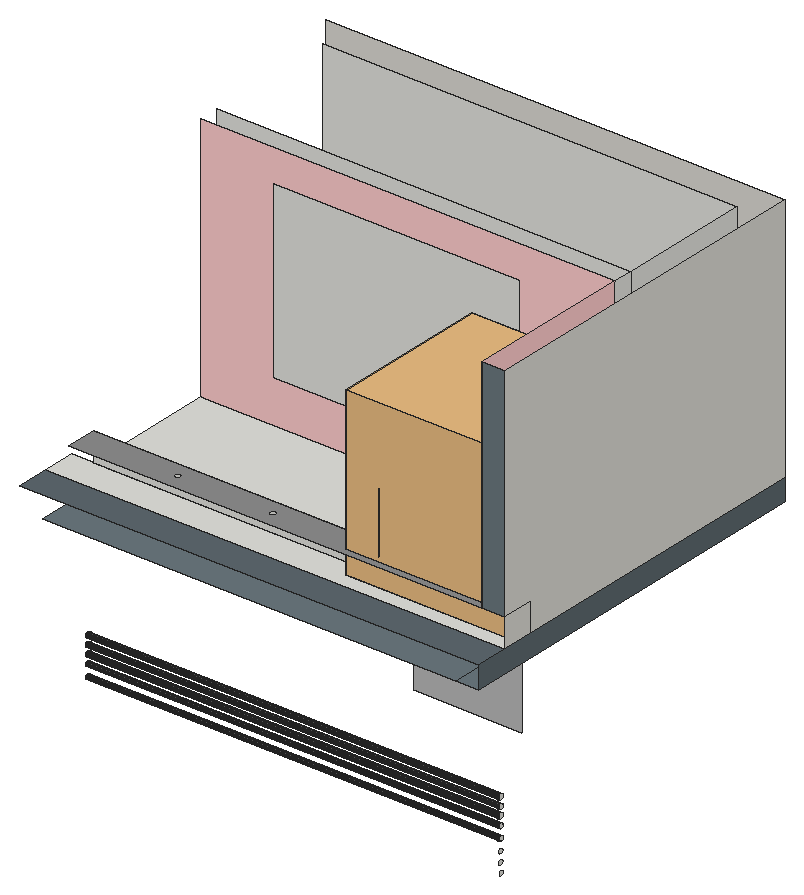
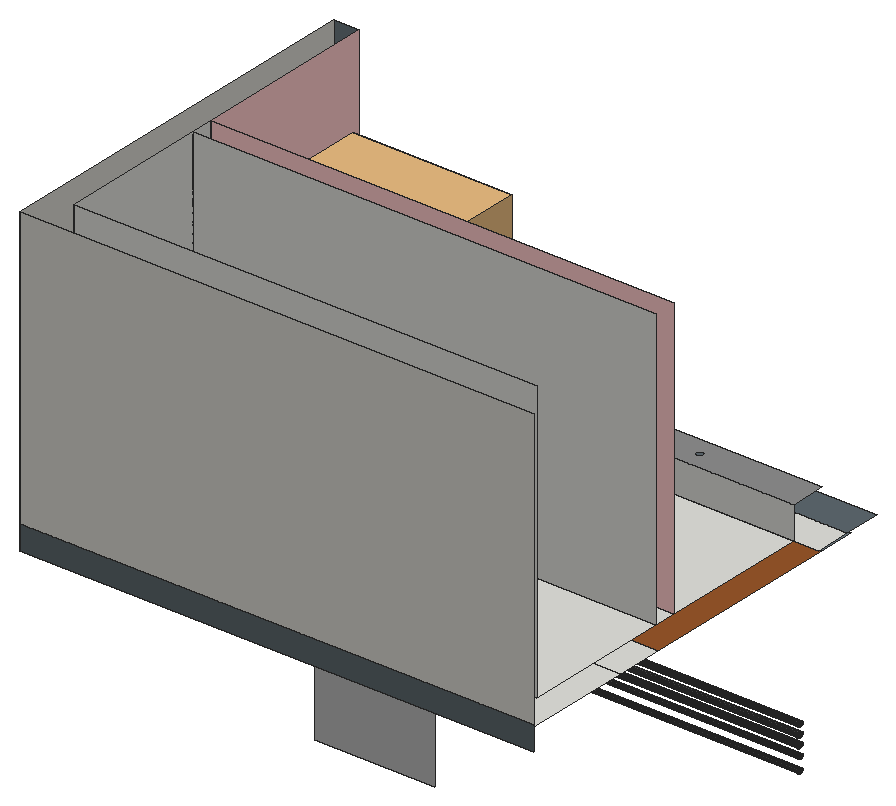
# SketchUp Ruby script. Lengths in inches.
U = 1.inch
M = Sketchup.active_model
def pt(a) = Geom::Point3d.new(a.map { |v| v * U })
def face(e, loops, mat)
  f = e.add_face(loops[0].map { |a| pt(a) })
  loops[1..].each { |l| e.add_face(l.map { |a| pt(a) }).erase! }
  f.material = f.back_material = mat if mat
  f
end
# faces: each face lists its corners as indices into pts; further lists are holes
def faces(e, pts, list, mat = nil) = list.each { |f| face(e, (f[0].is_a?(Array) ? f : [f]).map { |l| l.map { |i| pts[i] } }, mat) }
# xy, xz, yz: faces in a plane at the given z, y or x. An outline is a flat list of corners, or four numbers for a rectangle; further outlines are holes
def ring(l) = l.size == 4 ? [[l[0], l[1]], [l[2], l[1]], [l[2], l[3]], [l[0], l[3]]] : l.each_slice(2).to_a
def flat(e, list, mat, &to3) = list.each { |f| face(e, (f[0].is_a?(Array) ? f : [f]).map { |l| ring(l).map { |u, v| to3.(u, v) } }, mat) }
def xy(e, z, list, mat = nil) = flat(e, list, mat) { |x, y| [x, y, z] }
def xz(e, y, list, mat = nil) = flat(e, list, mat) { |x, z| [x, y, z] }
def yz(e, x, list, mat = nil) = flat(e, list, mat) { |y, z| [x, y, z] }
def lines(e, pts, list) = list.each { |a, b| e.add_line(pt(pts[a]), pt(pts[b])) }
# prism: a flat outline (further loops are holes) pulled along v
def prism(e, loops, v, mat = nil)
  f = face(e, loops, mat); d = Geom::Vector3d.new(v.map { |x| x * U })
  f.pushpull(f.normal.samedirection?(d) ? d.length : -d.length)
end
def box(e, o, s, mat = nil) = prism(e, [[o, [o[0] + s[0], o[1], o[2]], [o[0] + s[0], o[1] + s[1], o[2]], [o[0], o[1] + s[1], o[2]]]], [0, 0, s[2]], mat)
def at(x, y, z, deg = 0) = Geom::Transformation.translation(pt([x, y, z])) * Geom::Transformation.rotation(ORIGIN, Z_AXIS, deg.degrees)
def axes(o, x, y, z) = Geom::Transformation.new([*x, 0, *y, 0, *z, 0, *pt(o).to_a, 1])
def part(name) = M.definitions.add(name)
# library, detail: a bought-in or finely detailed component or shape, given as its bounding box
def library(name, o, s) = part(name).tap { |d| box(d.entities, o, s) }
def detail(e, o, s) = box(e.add_group.entities, o, s)
def put(e, d, t, mat = nil) = e.add_instance(d, t).tap { |i| i.material = mat if mat }
def group(e, t, mat = nil) = e.add_group.tap { |g| g.transformation = t; g.material = mat if mat }.entities
root = M.entities
M.materials.add("[Color A01]").color = [255, 204, 204]
M.materials.add("[Color M04]").color = [142, 142, 142]
M.materials.add("[Color M06]").color = [86, 86, 86]
M.materials.add("[Formica Speckled Grey]").color = [107, 120, 127]
M.materials.add("[Formica Speckled Grey]1").color = [94, 105, 111]
M.materials.add("[Mirror 01]").color = [185, 185, 185]
M.materials.add("[Terrazzo Tile Light]").color = [219, 217, 210]
M.materials.add("[Wood Cherry Original]").color = [152, 86, 42]
c1 = library("chau cay",[-24.34,-109.24,0],[56.46,62.58,79.69])
xy(root,157.1875,[[166.51,84,166.7,84.02,166.88,84.1,167.04,84.22,167.16,84.375,167.23,84.55,167.26,84.75,167.23,84.94,167.16,85.125,167.04,85.28,166.88,85.4,166.7,85.47,166.51,85.5,166.32,85.47,166.13,85.4,165.98,85.28,165.86,85.125,165.79,84.94,165.76,84.75,165.79,84.55,165.86,84.375,165.98,84.22,166.13,84.1,166.32,84.02]])
xy(root,195.875,[[202.95,77.29,209.59,113.38],[178.6,91.72,177.43,92.01,176.375,92.59,175.51,93.43,174.88,94.46,174.55,95.62,174.52,96.83,174.81,98,175.4,99.06,176.24,99.93,177.27,100.55,178.43,100.89,179.64,100.91,180.81,100.62,181.87,100.04,182.74,99.2,183.36,98.16,183.69,97,183.72,95.8,183.43,94.625,182.84,93.57,182.01,92.7,180.97,92.07,179.8125,91.74],[202.95,113.38,209.59,131.65],[80.125,131.65,202.95,143.96],[202.95,131.65,209.59,143.96],
  [80.125,143.96,202.95,174.55],[202.95,143.96,209.59,181.19]])
xy(root,195.875,[[80.125,67.6,202.95,77.29],[202.95,67.6,209.59,77.29]],"[Formica Speckled Grey]")
xy(root,195.875,[[[80.125,77.29,202.95,131.65],[178.6,91.72,179.8125,91.74,180.97,92.07,182.01,92.7,182.84,93.57,183.43,94.625,183.72,95.8,183.69,97,183.36,98.16,182.74,99.2,181.87,100.04,180.81,100.62,179.64,100.91,178.43,100.89,177.27,100.55,176.24,99.93,175.4,99.06,174.81,98,174.52,96.83,174.55,95.62,174.88,94.46,175.51,93.43,176.375,92.59,177.43,92.01],[137.04,91.72,138.25,91.74,139.41,92.07,140.44,92.7,141.28,93.57,141.86,94.625,142.15,95.8,142.13,97,141.8,98.16,141.17,99.2,140.3,100.04,139.25,100.62,138.07,100.91,136.87,100.89,135.71,100.55,134.67,99.93,133.84,99.06,133.25,98,132.96,96.83,132.98,95.62,133.32,94.46,133.94,93.43,134.8125,92.59,135.87,92.01],[102.79,91.72,104,91.74,105.16,92.07,106.19,92.7,107.03,93.57,107.61,94.625,107.9,95.8,107.88,97,107.55,98.16,106.92,99.2,106.05,100.04,105,100.62,103.82,100.91,102.62,100.89,101.46,100.55,100.42,99.93,99.59,99.06,99,98,98.71,96.83,98.73,95.62,99.07,94.46,99.69,93.43,100.5625,92.59,101.62,92.01]]],"[Wood Cherry Original]")
xy(root,202.375,[[73.48,77.29,209.59,86.77],[80.125,86.77,202.95,126.48],[80.125,126.48,202.95,132.38],[80.125,132.38,202.95,171.71]])
xy(root,202.375,[[73.48,67.6,209.59,77.29]],"[Formica Speckled Grey]1")
xy(root,210.9375,[[202.95,77.29,209.59,86.77],[169.66,81.17,169.4,81.21,169.16,81.31,168.95,81.46,168.8,81.67,168.7,81.91,168.66,82.17,168.7,82.43,168.8,82.67,168.95,82.88,169.16,83.04,169.4,83.14,169.66,83.17,169.92,83.14,170.16,83.04,170.37,82.88,170.53,82.67,170.625,82.43,170.66,82.17,170.625,81.91,170.53,81.67,170.37,81.46,170.16,81.31,169.92,81.21]])
xy(root,210.9375,[[[80.125,77.29,202.95,86.77],[108.66,81.17,108.4,81.21,108.16,81.31,107.95,81.46,107.8,81.67,107.7,81.91,107.66,82.17,107.7,82.43,107.8,82.67,107.95,82.88,108.16,83.04,108.4,83.14,108.66,83.17,108.92,83.14,109.16,83.04,109.37,82.88,109.53,82.67,109.625,82.43,109.66,82.17,109.625,81.91,109.53,81.67,109.37,81.46,109.16,81.31,108.92,81.21],[169.66,81.17,169.4,81.21,169.16,81.31,168.95,81.46,168.8,81.67,168.7,81.91,168.66,82.17,168.7,82.43,168.8,82.67,168.95,82.88,169.16,83.04,169.4,83.14,169.66,83.17,169.92,83.14,170.16,83.04,170.37,82.88,170.53,82.67,170.625,82.43,170.66,82.17,170.625,81.91,170.53,81.67,170.37,81.46,170.16,81.31,169.92,81.21],[136.97,81.17,136.71,81.21,136.47,81.31,136.27,81.46,136.11,81.67,136.01,81.91,135.97,82.17,136.01,82.43,136.11,82.67,136.27,82.88,136.47,83.04,136.71,83.14,136.97,83.17,137.23,83.14,137.47,83.04,137.68,82.88,137.84,82.67,137.9375,82.43,137.97,82.17,137.9375,81.91,137.84,81.67,137.68,81.46,137.47,81.31,137.23,81.21]]],"[Color M04]")
xz(root,77.29,[[202.95,210.9375,209.59,276.375]],"[Formica Speckled Grey]")
xz(root,86.77,[[80.125,202.375,202.95,210.9375],[202.95,202.375,209.59,210.9375]])
xz(root,126.48,[[[80.125,202.375,202.95,276.375],[101.56,215.09,174.81,266.84]]],"[Color A01]")
xz(root,131.65,[[139.18,142.9,171.11,185.91]],"[Mirror 01]")
xz(root,132.38,[[80.125,202.375,202.95,276.375]])
xz(root,171.71,[[80.125,202.375,202.95,276.375]])
xz(root,181.19,[[73.48,195.875,209.59,202.375]],"[Formica Speckled Grey]1")
xz(root,181.19,[[73.48,202.375,209.59,276.375]],"[Terrazzo Tile Light]")
yz(root,202.95,[[84.31,136.76,84.47,136.78,84.62,136.84,84.75,136.94,84.85,137.07,84.91,137.22,84.93,137.39,84.91,137.55,84.85,137.7,84.75,137.83,84.62,137.93,84.47,137.99,84.31,138.01,84.15,137.99,84,137.93,83.87,137.83,83.77,137.7,83.7,137.55,83.68,137.39,83.7,137.22,83.77,137.07,83.87,136.94,84,136.84,84.15,136.78],[84.14,139.71,84.3,139.73,84.45,139.79,84.58,139.89,84.68,140.02,84.74,140.17,84.77,140.33,84.74,140.49,84.68,140.64,84.58,140.77,84.45,140.87,84.3,140.93,84.14,140.96,83.98,140.93,83.83,140.87,83.7,140.77,83.6,140.64,83.54,140.49,83.52,140.33,83.54,140.17,83.6,140.02,83.7,139.89,83.83,139.79,83.98,139.73],[84.14,142.77,84.3,142.79,84.45,142.85,84.58,142.95,84.68,143.08,84.74,143.23,84.77,143.39,84.74,143.56,84.68,143.71,84.58,143.84,84.45,143.93,84.3,144,84.14,144.02,83.98,144,83.83,143.93,83.7,143.84,83.6,143.71,83.54,143.56,83.52,143.39,83.54,143.23,83.6,143.08,83.7,142.95,83.83,142.85,83.98,142.79],[84.31,145.95,84.47,145.97,84.62,146.03,84.75,146.13,84.85,146.26,84.91,146.41,84.93,146.57,84.91,146.74,84.85,146.89,84.75,147.02,84.62,147.11,84.47,147.18,84.31,147.2,84.15,147.18,84,147.11,83.87,147.02,83.77,146.89,83.7,146.74,83.68,146.57,83.7,146.41,83.77,146.26,83.87,146.13,84,146.03,84.15,145.97],[84.31,149.39,84.47,149.41,84.62,149.47,84.75,149.57,84.85,149.7,84.91,149.85,84.93,150.01,84.91,150.17,84.85,150.32,84.75,150.45,84.62,150.55,84.47,150.61,84.31,150.64,84.15,150.61,84,150.55,83.87,150.45,83.77,150.32,83.7,150.17,83.68,150.01,83.7,149.85,83.77,149.7,83.87,149.57,84,149.47,84.15,149.41],
  [84.34,151.97,84.51,152,84.68,152.06,84.82,152.17,84.93,152.32,85,152.48,85.02,152.66,85,152.84,84.93,153,84.82,153.15,84.68,153.26,84.51,153.32,84.34,153.35,84.16,153.32,83.99,153.26,83.85,153.15,83.74,153,83.67,152.84,83.65,152.66,83.67,152.48,83.74,152.32,83.85,152.17,83.99,152.06,84.16,152],[84.34,154.47,84.51,154.5,84.68,154.56,84.82,154.67,84.93,154.82,85,154.98,85.02,155.16,85,155.34,84.93,155.5,84.82,155.65,84.68,155.76,84.51,155.82,84.34,155.85,84.16,155.82,83.99,155.76,83.85,155.65,83.74,155.5,83.67,155.34,83.65,155.16,83.67,154.98,83.74,154.82,83.85,154.67,83.99,154.56,84.16,154.5],[84.34,157.04,84.51,157.06,84.68,157.13,84.82,157.24,84.93,157.38,85,157.54,85.02,157.72,85,157.9,84.93,158.07,84.82,158.21,84.68,158.32,84.51,158.39,84.34,158.41,84.16,158.39,83.99,158.32,83.85,158.21,83.74,158.07,83.67,157.9,83.65,157.72,83.67,157.54,83.74,157.38,83.85,157.24,83.99,157.13,84.16,157.06],[126.48,202.375,132.38,276.375],[132.38,202.375,171.71,276.375]])
yz(root,202.95,[[[86.77,202.375,86.77,210.9375,77.29,210.9375,77.29,276.375,126.48,276.375,126.48,202.375],[82.17,234.08,82.42,234.11,82.67,234.21,82.875,234.37,83.03,234.58,83.13,234.82,83.17,235.08,83.13,235.34,83.03,235.58,82.875,235.79,82.67,235.94,82.42,236.04,82.17,236.08,81.91,236.04,81.67,235.94,81.46,235.79,81.3,235.58,81.2,235.34,81.17,235.08,81.2,234.82,81.3,234.58,81.46,234.37,81.67,234.21,81.91,234.11],[82.38,211.9,82.55,211.92,82.7,211.98,82.83,212.08,82.92,212.21,82.99,212.36,83.01,212.52,82.99,212.68,82.92,212.83,82.83,212.96,82.7,213.0625,82.55,213.125,82.38,213.15,82.22,213.125,82.07,213.0625,81.94,212.96,81.84,212.83,81.78,212.68,81.76,212.52,81.78,212.36,81.84,212.21,81.94,212.08,82.07,211.98,82.22,211.92],[82.38,228.4,82.55,228.42,82.7,228.48,82.83,228.58,82.92,228.71,82.99,228.86,83.01,229.02,82.99,229.18,82.92,229.33,82.83,229.46,82.7,229.5625,82.55,229.625,82.38,229.65,82.22,229.625,82.07,229.5625,81.94,229.46,81.84,229.33,81.78,229.18,81.76,229.02,81.78,228.86,81.84,228.71,81.94,228.58,82.07,228.48,82.22,228.42],[82.38,217.52,82.55,217.54,82.7,217.61,82.83,217.71,82.92,217.83,82.99,217.99,83.01,218.15,82.99,218.31,82.92,218.46,82.83,218.59,82.7,218.6875,82.55,218.75,82.38,218.77,82.22,218.75,82.07,218.6875,81.94,218.59,81.84,218.46,81.78,218.31,81.76,218.15,81.78,217.99,81.84,217.83,81.94,217.71,82.07,217.61,82.22,217.54],[82.38,225.9,82.55,225.92,82.7,225.98,82.83,226.08,82.92,226.21,82.99,226.36,83.01,226.52,82.99,226.68,82.92,226.83,82.83,226.96,82.7,227.0625,82.55,227.125,82.38,227.15,82.22,227.125,82.07,227.0625,81.94,226.96,81.84,226.83,81.78,226.68,81.76,226.52,81.78,226.36,81.84,226.21,81.94,226.08,82.07,225.98,82.22,225.92],[82.38,220.46,82.55,220.48,82.7,220.54,82.83,220.64,82.92,220.77,82.99,220.92,83.01,221.08,82.99,221.25,82.92,221.4,82.83,221.53,82.7,221.625,82.55,221.6875,82.38,221.71,82.22,221.6875,82.07,221.625,81.94,221.53,81.84,221.4,81.78,221.25,81.76,221.08,81.78,220.92,81.84,220.77,81.94,220.64,82.07,220.54,82.22,220.48],[82.38,223.27,82.55,223.29,82.7,223.36,82.83,223.46,82.92,223.58,82.99,223.74,83.01,223.9,82.99,224.06,82.92,224.21,82.83,224.34,82.7,224.4375,82.55,224.5,82.38,224.52,82.22,224.5,82.07,224.4375,81.94,224.34,81.84,224.21,81.78,224.06,81.76,223.9,81.78,223.74,81.84,223.58,81.94,223.46,82.07,223.36,82.22,223.29],[82.38,214.83,82.55,214.86,82.7,214.92,82.83,215.02,82.92,215.15,82.99,215.3,83.01,215.46,82.99,215.62,82.92,215.77,82.83,215.9,82.7,216,82.55,216.0625,82.38,216.08,82.22,216.0625,82.07,216,81.94,215.9,81.84,215.77,81.78,215.62,81.76,215.46,81.78,215.3,81.84,215.15,81.94,215.02,82.07,214.92,82.22,214.86],[82.38,230.9,82.55,230.92,82.7,230.98,82.83,231.08,82.92,231.21,82.99,231.36,83.01,231.52,82.99,231.68,82.92,231.83,82.83,231.96,82.7,232.0625,82.55,232.125,82.38,232.15,82.22,232.125,82.07,232.0625,81.94,231.96,81.84,231.83,81.78,231.68,81.76,231.52,81.78,231.36,81.84,231.21,81.94,231.08,82.07,230.98,82.22,230.92]]],"[Color A01]")
yz(root,209.59,[[67.6,195.875,181.19,202.375]],"[Formica Speckled Grey]1")
yz(root,209.59,[[77.29,202.375,86.77,210.9375],[86.77,202.375,181.19,202.375,181.19,276.375,77.29,276.375,77.29,210.9375,86.77,210.9375]],"[Terrazzo Tile Light]")
p = [[202.95,84,146.03],[202.95,83.87,146.13],[80.125,83.87,146.13],[80.125,84,146.03],[202.95,84.15,145.97],[80.125,84.15,145.97],
  [202.95,84.62,146.03],[202.95,84.47,145.97],[80.125,84.47,145.97],[80.125,84.62,146.03],[202.95,84.75,146.13],[80.125,84.75,146.13],
  [202.95,83.77,146.26],[80.125,83.77,146.26],[202.95,84.85,146.26],[80.125,84.85,146.26],[202.95,83.7,146.41],[80.125,83.7,146.41],
  [202.95,84.91,146.41],[80.125,84.91,146.41],[202.95,83.68,146.57],[80.125,83.68,146.57],[202.95,84.93,146.57],[80.125,84.93,146.57],
  [202.95,83.7,146.74],[80.125,83.7,146.74],[202.95,84.91,146.74],[80.125,84.91,146.74],[202.95,83.77,146.89],[80.125,83.77,146.89],
  [202.95,84.85,146.89],[80.125,84.85,146.89],[202.95,83.87,147.02],[80.125,83.87,147.02],[202.95,84.75,147.02],[80.125,84.75,147.02],
  [202.95,84,147.11],[80.125,84,147.11],[202.95,84.62,147.11],[80.125,84.62,147.11],[202.95,84.15,147.18],[80.125,84.15,147.18],
  [202.95,84.47,147.18],[80.125,84.47,147.18],[202.95,84.31,147.2],[80.125,84.31,147.2],[202.95,84.15,149.41],[202.95,84,149.47],
  [80.125,84,149.47],[80.125,84.15,149.41],[202.95,84.31,149.39],[80.125,84.31,149.39],[202.95,84.47,149.41],[80.125,84.47,149.41],
  [202.95,84.62,149.47],[80.125,84.62,149.47],[202.95,83.87,149.57],[80.125,83.87,149.57],[202.95,84.75,149.57],[80.125,84.75,149.57],
  [202.95,83.77,149.7],[80.125,83.77,149.7],[202.95,84.85,149.7],[80.125,84.85,149.7],[202.95,83.7,149.85],[80.125,83.7,149.85],
  [202.95,84.91,149.85],[80.125,84.91,149.85],[202.95,83.68,150.01],[80.125,83.68,150.01],[202.95,84.93,150.01],[80.125,84.93,150.01],
  [202.95,83.7,150.17],[80.125,83.7,150.17],[202.95,84.91,150.17],[80.125,84.91,150.17],[202.95,83.77,150.32],[80.125,83.77,150.32],
  [202.95,84.85,150.32],[80.125,84.85,150.32],[202.95,83.87,150.45],[80.125,83.87,150.45],[202.95,84.75,150.45],[80.125,84.75,150.45],
  [202.95,84,150.55],[80.125,84,150.55],[202.95,84.62,150.55],[80.125,84.62,150.55],[202.95,84.15,150.61],[80.125,84.15,150.61],
  [202.95,84.31,150.64],[80.125,84.31,150.64],[202.95,84.47,150.61],[80.125,84.47,150.61],[202.95,84.16,152],[202.95,83.99,152.06],
  [80.125,83.99,152.06],[80.125,84.16,152],[202.95,84.34,151.97],[80.125,84.34,151.97],[202.95,84.51,152],[80.125,84.51,152],
  [202.95,84.68,152.06],[80.125,84.68,152.06],[202.95,83.85,152.17],[80.125,83.85,152.17],[202.95,84.82,152.17],[80.125,84.82,152.17],
  [202.95,83.74,152.32],[80.125,83.74,152.32],[202.95,84.93,152.32],[80.125,84.93,152.32],[202.95,83.67,152.48],[80.125,83.67,152.48],
  [202.95,85,152.48],[80.125,85,152.48],[202.95,83.65,152.66],[80.125,83.65,152.66],[202.95,85.02,152.66],[80.125,85.02,152.66],
  [202.95,83.67,152.84],[80.125,83.67,152.84],[202.95,85,152.84],[80.125,85,152.84],[202.95,83.74,153],[80.125,83.74,153],
  [202.95,84.93,153],[80.125,84.93,153],[202.95,83.85,153.15],[80.125,83.85,153.15],[202.95,84.82,153.15],[80.125,84.82,153.15],
  [202.95,83.99,153.26],[80.125,83.99,153.26],[202.95,84.68,153.26],[80.125,84.68,153.26],[202.95,84.16,153.32],[80.125,84.16,153.32],
  [202.95,84.34,153.35],[80.125,84.34,153.35],[202.95,84.51,153.32],[80.125,84.51,153.32],[202.95,84.16,154.5],[202.95,83.99,154.56],
  [80.125,83.99,154.56],[80.125,84.16,154.5],[202.95,84.34,154.47],[80.125,84.34,154.47],[202.95,84.51,154.5],[80.125,84.51,154.5],
  [202.95,84.68,154.56],[80.125,84.68,154.56],[202.95,83.85,154.67],[80.125,83.85,154.67],[202.95,84.82,154.67],[80.125,84.82,154.67],
  [202.95,83.74,154.82],[80.125,83.74,154.82],[202.95,84.93,154.82],[80.125,84.93,154.82],[202.95,83.67,154.98],[80.125,83.67,154.98],
  [202.95,85,154.98],[80.125,85,154.98],[202.95,83.65,155.16],[80.125,83.65,155.16],[202.95,85.02,155.16],[80.125,85.02,155.16],
  [202.95,83.67,155.34],[80.125,83.67,155.34],[202.95,85,155.34],[80.125,85,155.34],[202.95,83.74,155.5],[80.125,83.74,155.5],
  [202.95,84.93,155.5],[80.125,84.93,155.5],[202.95,83.85,155.65],[80.125,83.85,155.65],[202.95,84.82,155.65],[80.125,84.82,155.65],
  [202.95,83.99,155.76],[80.125,83.99,155.76],[202.95,84.68,155.76],[80.125,84.68,155.76],[202.95,84.16,155.82],[80.125,84.16,155.82],
  [202.95,84.34,155.85],[80.125,84.34,155.85],[202.95,84.51,155.82],[80.125,84.51,155.82],[202.95,84.34,157.04],[202.95,84.16,157.06],
  [80.125,84.16,157.06],[80.125,84.34,157.04],[202.95,84.51,157.06],[80.125,84.51,157.06],[202.95,83.99,157.13],[202.95,83.85,157.24],
  [80.125,83.85,157.24],[80.125,83.99,157.13],[202.95,84.68,157.13],[80.125,84.68,157.13],[202.95,84.82,157.24],[80.125,84.82,157.24],
  [202.95,83.74,157.38],[80.125,83.74,157.38],[202.95,83.67,157.54],[80.125,83.67,157.54],[202.95,83.65,157.72],[80.125,83.65,157.72],
  [202.95,85.02,157.72],[202.95,85,157.54],[80.125,85,157.54],[80.125,85.02,157.72],[202.95,83.67,157.9],[80.125,83.67,157.9],
  [202.95,85,157.9],[80.125,85,157.9],[202.95,83.74,158.07],[80.125,83.74,158.07],[202.95,84.93,158.07],[80.125,84.93,158.07],
  [202.95,83.85,158.21],[80.125,83.85,158.21],[202.95,84.82,158.21],[80.125,84.82,158.21],[202.95,83.99,158.32],[80.125,83.99,158.32],
  [202.95,84.68,158.32],[80.125,84.68,158.32],[202.95,84.16,158.39],[80.125,84.16,158.39],[202.95,84.51,158.39],[80.125,84.51,158.39],
  [202.95,84.34,158.41],[80.125,84.34,158.41],[169.16,81.31,210.9375],[169.4,81.21,210.9375],[169.4,81.21,234.625],[169.16,81.31,234.625],
  [169.66,81.17,210.9375],[169.66,81.17,234.625],[169.92,81.21,210.9375],[169.92,81.21,234.625],[170.16,81.31,210.9375],[170.16,81.31,234.625],
  [168.95,81.46,210.9375],[168.95,81.46,234.625],[170.37,81.46,210.9375],[170.37,81.46,234.625],[168.8,81.67,210.9375],[168.8,81.67,234.625],
  [170.53,81.67,210.9375],[170.53,81.67,234.625],[168.7,81.91,210.9375],[168.7,81.91,234.625],[170.625,81.91,210.9375],[170.625,81.91,234.625],
  [168.66,82.17,210.9375],[168.66,82.17,234.625],[170.66,82.17,210.9375],[170.66,82.17,234.625],[168.7,82.43,210.9375],[168.7,82.43,234.625],
  [170.625,82.43,210.9375],[170.625,82.43,234.625],[168.8,82.67,210.9375],[168.8,82.67,234.625],[170.53,82.67,210.9375],[170.53,82.67,234.625],
  [168.95,82.88,210.9375],[168.95,82.88,234.625],[170.37,82.88,210.9375],[170.37,82.88,234.625],[169.16,83.04,210.9375],[169.16,83.04,234.625],
  [170.16,83.04,210.9375],[170.16,83.04,234.625],[169.4,83.14,210.9375],[169.4,83.14,234.625],[169.92,83.14,210.9375],[169.92,83.14,234.625],
  [169.66,83.17,210.9375],[169.66,83.17,234.625]]
faces(root,p,[[0,1,2,3],[4,0,3,5],[6,7,8,9],[10,6,9,11],[1,12,13,2],[14,10,11,15],[12,16,17,13],[18,14,15,19],
  [16,20,21,17],[22,18,19,23],[20,24,25,21],[26,22,23,27],[24,28,29,25],[30,26,27,31],[28,32,33,29],[34,30,31,35],
  [32,36,37,33],[38,34,35,39],[36,40,41,37],[42,38,39,43],[40,44,45,41],[44,42,43,45],[46,47,48,49],[50,46,49,51],
  [52,50,51,53],[54,52,53,55],[47,56,57,48],[58,54,55,59],[56,60,61,57],[62,58,59,63],[60,64,65,61],[66,62,63,67],
  [64,68,69,65],[70,66,67,71],[68,72,73,69],[74,70,71,75],[72,76,77,73],[78,74,75,79],[76,80,81,77],[82,78,79,83],
  [80,84,85,81],[86,82,83,87],[84,88,89,85],[88,90,91,89],[90,92,93,91],[92,86,87,93],[94,95,96,97],[98,94,97,99],
  [100,98,99,101],[102,100,101,103],[95,104,105,96],[106,102,103,107],[104,108,109,105],[110,106,107,111],[108,112,113,109],[114,110,111,115],
  [112,116,117,113],[118,114,115,119],[116,120,121,117],[122,118,119,123],[120,124,125,121],[126,122,123,127],[124,128,129,125],[130,126,127,131],
  [128,132,133,129],[134,130,131,135],[132,136,137,133],[136,138,139,137],[138,140,141,139],[140,134,135,141],[142,143,144,145],[146,142,145,147],
  [148,146,147,149],[150,148,149,151],[143,152,153,144],[154,150,151,155],[152,156,157,153],[158,154,155,159],[156,160,161,157],[162,158,159,163],
  [160,164,165,161],[166,162,163,167],[164,168,169,165],[170,166,167,171],[168,172,173,169],[174,170,171,175],[172,176,177,173],[178,174,175,179],
  [176,180,181,177],[182,178,179,183],[180,184,185,181],[184,186,187,185],[186,188,189,187],[188,182,183,189],[190,191,192,193],[194,190,193,195],
  [196,197,198,199],[191,196,199,192],[200,194,195,201],[202,200,201,203],[197,204,205,198],[204,206,207,205],[206,208,209,207],[210,211,212,213],
  [208,214,215,209],[216,210,213,217],[214,218,219,215],[220,216,217,221],[218,222,223,219],[224,220,221,225],[222,226,227,223],[228,224,225,229],
  [226,230,231,227],[232,228,229,233],[230,234,235,231],[234,232,233,235],[236,237,238,239],[237,240,241,238],[240,242,243,241],[242,244,245,243],
  [246,236,239,247],[244,248,249,245],[250,246,247,251],[248,252,253,249],[254,250,251,255],[252,256,257,253],[258,254,255,259],[256,260,261,257],
  [262,258,259,263],[260,264,265,261],[266,262,263,267],[264,268,269,265],[270,266,267,271],[268,272,273,269],[274,270,271,275],[272,276,277,273],
  [278,274,275,279],[276,280,281,277],[282,278,279,283],[280,282,283,281]],"[Color M06]")
put(root,c1,axes([181.56,161.48,204.11],[0.86,0,0],[0,0.75,0],[0,0,0.615]))
